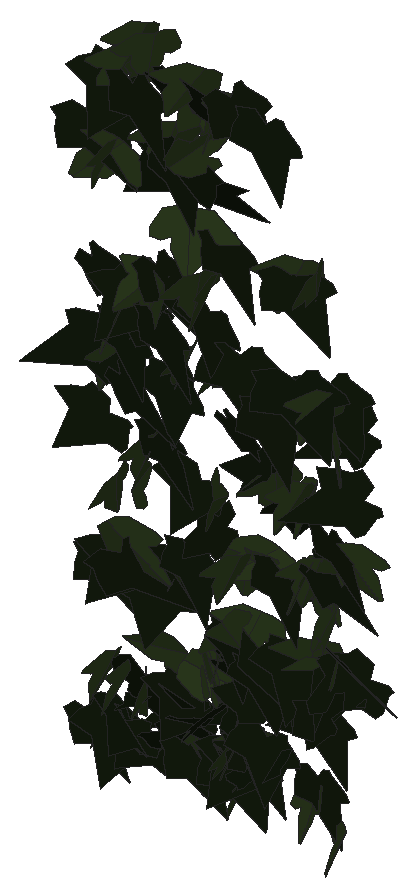
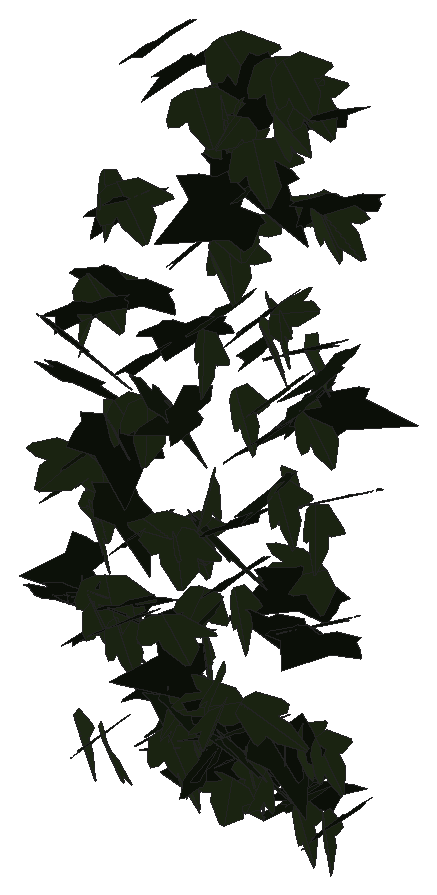
# SketchUp Ruby script. Lengths in inches.
U = 1.inch
M = Sketchup.active_model
def pt(a) = Geom::Point3d.new(a.map { |v| v * U })
def face(e, loops, mat)
  f = e.add_face(loops[0].map { |a| pt(a) })
  loops[1..].each { |l| e.add_face(l.map { |a| pt(a) }).erase! }
  f.material = f.back_material = mat if mat
  f
end
# faces: each face lists its corners as indices into pts; further lists are holes
def faces(e, pts, list, mat = nil) = list.each { |f| face(e, (f[0].is_a?(Array) ? f : [f]).map { |l| l.map { |i| pts[i] } }, mat) }
# xy, xz, yz: faces in a plane at the given z, y or x. An outline is a flat list of corners, or four numbers for a rectangle; further outlines are holes
def ring(l) = l.size == 4 ? [[l[0], l[1]], [l[2], l[1]], [l[2], l[3]], [l[0], l[3]]] : l.each_slice(2).to_a
def flat(e, list, mat, &to3) = list.each { |f| face(e, (f[0].is_a?(Array) ? f : [f]).map { |l| ring(l).map { |u, v| to3.(u, v) } }, mat) }
def xy(e, z, list, mat = nil) = flat(e, list, mat) { |x, y| [x, y, z] }
def xz(e, y, list, mat = nil) = flat(e, list, mat) { |x, z| [x, y, z] }
def yz(e, x, list, mat = nil) = flat(e, list, mat) { |y, z| [x, y, z] }
def lines(e, pts, list) = list.each { |a, b| e.add_line(pt(pts[a]), pt(pts[b])) }
# prism: a flat outline (further loops are holes) pulled along v
def prism(e, loops, v, mat = nil)
  f = face(e, loops, mat); d = Geom::Vector3d.new(v.map { |x| x * U })
  f.pushpull(f.normal.samedirection?(d) ? d.length : -d.length)
end
def box(e, o, s, mat = nil) = prism(e, [[o, [o[0] + s[0], o[1], o[2]], [o[0] + s[0], o[1] + s[1], o[2]], [o[0], o[1] + s[1], o[2]]]], [0, 0, s[2]], mat)
def at(x, y, z, deg = 0) = Geom::Transformation.translation(pt([x, y, z])) * Geom::Transformation.rotation(ORIGIN, Z_AXIS, deg.degrees)
def axes(o, x, y, z) = Geom::Transformation.new([*x, 0, *y, 0, *z, 0, *pt(o).to_a, 1])
def part(name) = M.definitions.add(name)
# library, detail: a bought-in or finely detailed component or shape, given as its bounding box
def library(name, o, s) = part(name).tap { |d| box(d.entities, o, s) }
def detail(e, o, s) = box(e.add_group.entities, o, s)
def put(e, d, t, mat = nil) = e.add_instance(d, t).tap { |i| i.material = mat if mat }
def group(e, t, mat = nil) = e.add_group.tap { |g| g.transformation = t; g.material = mat if mat }.entities
root = M.entities
M.materials.add("1026 AP 7946 SUNNY SIDE UP").color = [254, 231, 186]
M.materials.add("efeu1").color = [18, 25, 13]
M.materials.add("efeu2").color = [43, 57, 29]
c1 = part("ivyleaf_10")
p = [[0,0.5,-0.03],[-0.0625,2.02,-0.43],[-0.19,2.01,-0.46],[-0.54,1.05,-0.29],[-0.52,0.625,-0.18],[-0.83,0.76,-0.28],
  [-1.16,0.64,-0.33],[-1.15,0.33,-0.24],[-0.77,-0.39,0.02],[-0.3,-0.51,0.16],[0.04,-0.48,0.23],[-0.02,2.01,-0.4375],
  [-0.06,2.01,-0.43],[0.04,-0.49,0.23],[0.67,-0.49,0.14],[1.38,0.36,-0.2],[1.375,0.51,-0.24],[0.81,0.65,-0.19],
  [0.62,0.59,-0.15],[0.6,1.09,-0.28],[0.5,1.23,-0.31]]
faces(c1.entities,p,[[0,1,2,3,4,5,6,7,8,9,10],[11,12,0,13,14,15,16,17,18,19,20]],"efeu2")
c2 = part("ivyleaf_9")
p = [[1.54,2.16,1.25],[1.36,2.04,1.19],[-0.21,0.99,0.68],[-0.71,1.11,0.82],[-0.85,0.86,0.67],[-0.8,0.17,0.21],
  [-0.9,-0.01,0.1],[-0.67,-0.16,-0.02],[-0.08,-0.08,-0.05],[-0.03,-0.6,-0.4],[0.65,-0.88,-0.66],[0.83,-0.6,-0.49],
  [1.29,-0.42,-0.43],[1.8125,-0.07,-0.26],[1.21,0.44,0.15]]
faces(c2.entities,p,[[0,1,2,3,4,5,6,7,8,9,10,11,12,13,14]],"efeu1")
put(root,c1,axes([118.05,212.21,283.12],[-0.37131,0.05928,-0.28207],[0.39687,-0.11138,-0.24944],[-0.19234,-0.34425,0.02985]),"1026 AP 7946 SUNNY SIDE UP")
put(root,c2,axes([120.52,212.35,290.41],[0.01109,-0.35714,0.01681],[0.00161,-0.01832,-0.3681],[0.5623,0.00709,0.00072]),"1026 AP 7946 SUNNY SIDE UP")
put(root,c2,axes([120.52,212.35,280.61],[-0.10934,-0.30959,0.0089],[0.00379,-0.01119,-0.32692],[0.48707,-0.06941,0.00454]),"1026 AP 7946 SUNNY SIDE UP")
put(root,c2,axes([118.19,212.31,290.27],[0.13676,-0.35584,-0.02894],[-0.02006,0.02372,-0.37717],[0.56066,0.08765,-0.00644]),"1026 AP 7946 SUNNY SIDE UP")
put(root,c2,axes([117.93,212.4,279.95],[-0.28564,-0.27357,0.00365],[0.01734,-0.01343,-0.33795],[0.42988,-0.18123,0.01606]),"1026 AP 7946 SUNNY SIDE UP")
put(root,c1,axes([121.47,212.29,283.74],[-0.19698,-0.3026,0.06518],[-0.00906,-0.06782,-0.33715],[0.48657,-0.12376,0.02011]),"1026 AP 7946 SUNNY SIDE UP")
put(root,c1,axes([117.95,212.17,283.95],[-0.02269,-0.3263,-0.12185],[0.03595,0.11538,-0.33537],[0.54358,-0.02125,0.01709]),"1026 AP 7946 SUNNY SIDE UP")
put(root,c2,axes([118.17,212.11,282.84],[-0.00464,-0.10566,-0.34058],[0.18482,0.31014,-0.10157],[0.51254,-0.11279,0.03354]),"1026 AP 7946 SUNNY SIDE UP")
put(root,c2,axes([118.06,212.22,285.61],[0.32092,-0.25295,-0.1119],[-0.07031,0.10116,-0.33306],[0.42622,0.20714,0.02932]),"1026 AP 7946 SUNNY SIDE UP")
put(root,c2,axes([117.92,212.5,279.96],[-0.12651,-0.20876,0.23158],[-0.01217,-0.23213,-0.22511],[0.48358,-0.06046,0.05492]),"1026 AP 7946 SUNNY SIDE UP")
put(root,c2,axes([117.8,212.5,290.2],[-0.26607,-0.29238,0.1123],[-0.03521,-0.11418,-0.34671],[0.49031,-0.16686,0.03604]),"1026 AP 7946 SUNNY SIDE UP")
put(root,c2,axes([120.38,212.46,281.5],[-0.05446,-0.29507,0.12324],[0.13746,-0.12612,-0.29108],[0.48245,0.00263,0.09684]),"1026 AP 7946 SUNNY SIDE UP")
put(root,c2,axes([121.09,212.31,286.52],[-0.23251,-0.21185,-0.2599],[0.27253,0.18359,-0.26367],[0.43881,-0.22627,0.02605]),"1026 AP 7946 SUNNY SIDE UP")
put(root,c1,axes([119.45,212.4,287.52],[0.17888,-0.30544,0.1209],[0.04904,-0.1154,-0.33629],[0.51316,0.1175,-0.01]),"1026 AP 7946 SUNNY SIDE UP")
put(root,c1,axes([119.35,212.27,287.6],[-0.16301,-0.33822,-0.0361],[0.0191,0.03091,-0.36424],[0.53402,-0.10435,0.00201]),"1026 AP 7946 SUNNY SIDE UP")
put(root,c1,axes([121.22,212.41,283.57],[0.22591,-0.28506,0.12289],[0.04543,-0.12037,-0.32842],[0.48476,0.14412,-0.02649]),"1026 AP 7946 SUNNY SIDE UP")
put(root,c2,axes([120.6875,212.2,281.27],[-0.45565,-0.12997,0.10381],[0.12293,0.07243,0.32589],[-0.22831,0.29838,-0.03171]),"1026 AP 7946 SUNNY SIDE UP")
put(root,c1,axes([118.5,212.03,284.1],[0.02789,0.02027,0.34666],[-0.25633,0.29534,-0.00775],[-0.46377,-0.16201,0.02514]),"1026 AP 7946 SUNNY SIDE UP")
put(root,c1,axes([119.85,212.34,280.21],[0.09913,-0.30719,0.03282],[0.0014,-0.03412,-0.3232],[0.4859,0.06277,-0.00576]),"1026 AP 7946 SUNNY SIDE UP")
put(root,c2,axes([118.55,212.42,286.56],[0.17204,-0.33683,0.03028],[-0.00069,-0.03304,-0.36488],[0.53191,0.1089,-0.01027]),"1026 AP 7946 SUNNY SIDE UP")
put(root,c2,axes([117.88,212.54,282.48],[-0.30473,-0.22241,0.14591],[-0.02827,-0.16569,-0.29175],[0.41471,-0.17472,0.08733]),"1026 AP 7946 SUNNY SIDE UP")
put(root,c1,axes([118.23,212.55,287.1],[-0.12916,-0.07452,0.33716],[0.07859,-0.3363,-0.06785],[0.52256,0.03216,0.09354]),"1026 AP 7946 SUNNY SIDE UP")
put(root,c2,axes([117.53,212.54,285.94],[-0.01771,-0.10315,-0.36011],[-0.06862,-0.34623,0.10486],[-0.56806,0.04504,-0.00144]),"1026 AP 7946 SUNNY SIDE UP")
put(root,c1,axes([117.79,212.46,286.57],[0.26822,-0.26198,0.14637],[0.08507,-0.1355,-0.32174],[0.46198,0.17705,-0.02574]),"1026 AP 7946 SUNNY SIDE UP")
put(root,c1,axes([121.51,212.43,286.33],[-0.1676,-0.29899,0.14176],[-0.0358,-0.13938,-0.32694],[0.51742,-0.10649,0.0233]),"1026 AP 7946 SUNNY SIDE UP")
put(root,c1,axes([121.84,212.33,279.47],[0.18775,-0.30329,-0.03799],[-0.02193,0.03229,-0.3356],[0.47958,0.12021,-0.00047]),"1026 AP 7946 SUNNY SIDE UP")
put(root,c1,axes([119.2,212.44,290.74],[-0.25116,-0.28206,0.15218],[-0.09781,-0.13627,-0.33451],[0.49221,-0.171,0.01118]),"1026 AP 7946 SUNNY SIDE UP")
put(root,c2,axes([120.53,212.09,280.15],[0.14214,0.19395,0.24319],[-0.13834,0.25126,-0.17733],[-0.45865,-0.01568,0.12885]),"1026 AP 7946 SUNNY SIDE UP")
put(root,c1,axes([119.91,212.41,283.19],[-0.09981,-0.31758,0.06962],[-0.01095,-0.06934,-0.33398],[0.51102,-0.06351,0.00644]),"1026 AP 7946 SUNNY SIDE UP")
put(root,c2,axes([121.43,212.46,281.25],[0.05065,-0.32039,-0.03634],[0.01408,0.0345,-0.33128],[0.50632,0.03109,0.01285]),"1026 AP 7946 SUNNY SIDE UP")
put(root,c2,axes([119.77,212.57,281.8],[0.01605,-0.28926,0.16113],[0.04146,-0.15691,-0.2985],[0.51664,0.02158,0.01895]),"1026 AP 7946 SUNNY SIDE UP")
put(root,c1,axes([117.87,212.51,280.7],[0.09436,-0.26665,0.18193],[0.04982,-0.17539,-0.28252],[0.50175,0.06756,-0.00616]),"1026 AP 7946 SUNNY SIDE UP")
put(root,c2,axes([118.51,212.49,282.375],[-0.36498,-0.20044,-0.10045],[0.14258,0.0419,-0.31453],[0.31933,-0.24781,0.02563]),"1026 AP 7946 SUNNY SIDE UP")
put(root,c2,axes([119.13,212.39,279.96],[0.07979,-0.29118,-0.12477],[0.01211,0.12211,-0.30256],[0.49474,0.04397,0.02753]),"1026 AP 7946 SUNNY SIDE UP")
put(root,c1,axes([117.89,212.5,290.56],[-0.14815,-0.31006,0.15971],[-0.01477,-0.16012,-0.33296],[0.54613,-0.08844,0.03432]),"1026 AP 7946 SUNNY SIDE UP")
put(root,c2,axes([118.13,212.625,279.68],[-0.22099,-0.19114,0.22388],[-0.00666,-0.24129,-0.22177],[0.45632,-0.09609,0.10519]),"1026 AP 7946 SUNNY SIDE UP")
put(root,c2,axes([117.43,212.64,284.62],[-0.34331,-0.18123,0.17849],[-0.07273,-0.19794,-0.27289],[0.38862,-0.19715,0.10661]),"1026 AP 7946 SUNNY SIDE UP")
put(root,c2,axes([121.65,212.32,281.36],[-0.36437,0.21519,0.07506],[-0.09765,0.03829,-0.32525],[-0.343,-0.2395,0.01287]),"1026 AP 7946 SUNNY SIDE UP")
put(root,c1,axes([119.88,212.36,280.22],[0.16901,-0.28456,-0.0873],[-0.03486,0.08046,-0.3128],[0.46484,0.1095,0.00828]),"1026 AP 7946 SUNNY SIDE UP")
put(root,c2,axes([120.47,212.52,285.73],[0.00989,-0.34242,-0.0257],[0.00813,0.0231,-0.35263],[0.53957,0.00593,0.00579]),"1026 AP 7946 SUNNY SIDE UP")
put(root,c2,axes([118.91,212.65,280.59],[-0.24373,-0.23521,0.16587],[0.01614,-0.18915,-0.27332],[0.44909,-0.12085,0.09984]),"1026 AP 7946 SUNNY SIDE UP")
put(root,c2,axes([119.98,212.62,280.01],[-0.32822,-0.22991,0.08729],[-0.03143,-0.09664,-0.31658],[0.38472,-0.20405,0.0486]),"1026 AP 7946 SUNNY SIDE UP")
put(root,c1,axes([120.97,212.52,284.66],[-0.0809,-0.29893,0.14154],[-0.00747,-0.14008,-0.31279],[0.51837,-0.04867,0.01758]),"1026 AP 7946 SUNNY SIDE UP")
put(root,c1,axes([121.62,212.48,285.84],[-0.19204,0.26135,-0.17964],[0.07175,-0.17195,-0.29691],[-0.4901,-0.12758,0.02693]),"1026 AP 7946 SUNNY SIDE UP")
put(root,c2,axes([122.08,212.51,284.92],[-0.50167,0.02603,0.08828],[-0.13906,-0.04512,-0.32593],[-0.02073,-0.32722,0.05]),"1026 AP 7946 SUNNY SIDE UP")
put(root,c2,axes([121.45,212.36,283.69],[0.32651,-0.24493,-0.15128],[-0.07267,0.14864,-0.32496],[0.44198,0.20537,0.05832]),"1026 AP 7946 SUNNY SIDE UP")
put(root,c2,axes([118,212.68,286.68],[-0.32088,-0.22723,0.1565],[-0.04082,-0.17412,-0.3027],[0.42899,-0.18654,0.08826]),"1026 AP 7946 SUNNY SIDE UP")
put(root,c2,axes([119.84,212.53,279.92],[-0.09534,-0.29169,-0.1099],[0.22305,0.06906,-0.28154],[0.43346,-0.09969,0.1207]),"1026 AP 7946 SUNNY SIDE UP")
put(root,c2,axes([119.57,212.42,280.72],[-0.16859,0.26976,-0.13114],[0.05992,-0.12341,-0.29962],[-0.46623,-0.11341,0.00891]),"1026 AP 7946 SUNNY SIDE UP")
put(root,c2,axes([118.77,212.23,280.19],[0.35547,0.17185,0.17006],[0.22571,0.08173,-0.29142],[-0.29775,0.26712,-0.01789]),"1026 AP 7946 SUNNY SIDE UP")
put(root,c2,axes([119,212.6,282.91],[0.01702,-0.32559,0.01876],[-0.00312,-0.02014,-0.33571],[0.51292,0.01068,-0.00266]),"1026 AP 7946 SUNNY SIDE UP")
put(root,c2,axes([119.99,212.65,280.46],[0.02022,-0.30187,0.11982],[0.01947,-0.11757,-0.31187],[0.50927,0.01648,0.00717]),"1026 AP 7946 SUNNY SIDE UP")
put(root,c1,axes([121.55,212.4375,282.92],[0.29415,-0.31004,-0.09883],[-0.06089,0.08657,-0.37236],[0.50586,0.19071,0.01265]),"1026 AP 7946 SUNNY SIDE UP")
put(root,c1,axes([118.48,212.43,287.04],[0.30596,-0.26782,-0.10971],[-0.06688,0.09855,-0.33968],[0.44735,0.19791,0.02425]),"1026 AP 7946 SUNNY SIDE UP")
put(root,c1,axes([119.09,212.3,289.4],[-0.06176,-0.26401,0.26957],[0.10403,0.25549,0.27571],[-0.57684,0.07434,0.02086]),"1026 AP 7946 SUNNY SIDE UP")
put(root,c2,axes([121.47,212.59,284.05],[0.1858,-0.30234,0.05112],[0.02654,-0.04852,-0.33469],[0.48147,0.11935,-0.00128]),"1026 AP 7946 SUNNY SIDE UP")
put(root,c2,axes([118.66,212.67,288.98],[0.0436,-0.31457,0.13948],[0.06484,-0.13358,-0.32492],[0.53571,0.04177,0.02798]),"1026 AP 7946 SUNNY SIDE UP")
put(root,c1,axes([119.24,212.45,280.01],[-0.49317,0.02957,0.00586],[-0.01402,-0.03621,-0.32252],[-0.04517,-0.31159,0.03618]),"1026 AP 7946 SUNNY SIDE UP")
put(root,c1,axes([119.78,212.36,282.15],[-0.14789,-0.2643,-0.18328],[0.14948,0.15215,-0.28616],[0.47677,-0.12969,0.03287]),"1026 AP 7946 SUNNY SIDE UP")
put(root,c2,axes([117.24,212.49,279.83],[0.16529,-0.28242,-0.1147],[-0.03468,0.10871,-0.30936],[0.47515,0.10618,0.01732]),"1026 AP 7946 SUNNY SIDE UP")
put(root,c2,axes([119.88,212.5625,286.39],[-0.1336,-0.30921,-0.13611],[0.07399,0.12218,-0.32941],[0.52244,-0.09637,0.01184]),"1026 AP 7946 SUNNY SIDE UP")
put(root,c1,axes([117.52,212.58,280.76],[0.01132,-0.31376,0.08555],[0.01081,-0.08468,-0.32377],[0.51095,0.00874,0.00495]),"1026 AP 7946 SUNNY SIDE UP")
put(root,c1,axes([119.9375,212.55,279.66],[0.12837,-0.30126,0.03941],[0.00482,-0.04057,-0.32169],[0.47783,0.08134,-0.00735]),"1026 AP 7946 SUNNY SIDE UP")
put(root,c1,axes([118.26,212.43,280.63],[0.12111,-0.2841,-0.12206],[0.0374,0.12564,-0.29776],[0.48158,0.06169,0.05382]),"1026 AP 7946 SUNNY SIDE UP")
put(root,c2,axes([120.55,212.37,285.01],[-0.24553,0.28202,0.08284],[-0.09875,0.05498,-0.33056],[-0.44972,-0.16604,0.02736]),"1026 AP 7946 SUNNY SIDE UP")
put(root,c2,axes([119.21,212.72,286.8125],[-0.03955,-0.30964,0.13812],[0.02479,-0.13713,-0.31984],[0.53109,-0.01666,0.02522]),"1026 AP 7946 SUNNY SIDE UP")
put(root,c2,axes([120.08,212.58,280.24],[0.08954,-0.31135,-0.05016],[0.0424,0.05233,-0.3237],[0.49327,0.05202,0.03693]),"1026 AP 7946 SUNNY SIDE UP")
put(root,c1,axes([120.58,212.47,284.76],[-0.22333,-0.30352,-0.06918],[0.04765,0.05805,-0.34487],[0.48589,-0.1452,0.00203]),"1026 AP 7946 SUNNY SIDE UP")
put(root,c2,axes([117.92,212.61,280.49],[0.12649,-0.08318,0.31169],[0.33278,-0.21687,-0.12048],[0.36524,0.22641,0.00183]),"1026 AP 7946 SUNNY SIDE UP")
put(root,c2,axes([120.84,212.7,281.85],[-0.21586,-0.29723,0.02294],[0.02425,-0.03341,-0.33625],[0.46825,-0.13529,0.02799]),"1026 AP 7946 SUNNY SIDE UP")
put(root,c2,axes([118.58,212.5,290.42],[0.53033,-0.08673,0.09102],[0.12121,-0.05532,-0.35744],[0.15304,0.34437,-0.0323]),"1026 AP 7946 SUNNY SIDE UP")
put(root,c1,axes([117.53,212.61,288.96],[0.06499,-0.34102,0.04491],[-0.00603,-0.04631,-0.35403],[0.54095,0.04046,-0.00934]),"1026 AP 7946 SUNNY SIDE UP")
put(root,c1,axes([118.98,212.57,288.28],[0.45725,0.23068,-0.0269],[-0.00602,-0.03917,-0.38151],[-0.36522,0.28945,-0.02739]),"1026 AP 7946 SUNNY SIDE UP")
put(root,c2,axes([120.5,212.69,283.11],[0.04967,-0.33154,0.02036],[-0.01163,-0.02244,-0.34309],[0.52229,0.03103,-0.00958]),"1026 AP 7946 SUNNY SIDE UP")
put(root,c1,axes([117.61,212.54,288.97],[0.46329,0.03142,-0.19936],[-0.30853,0.043,-0.30004],[-0.00368,0.34997,0.05685]),"1026 AP 7946 SUNNY SIDE UP")
put(root,c2,axes([117.67,212.72,286.04],[0.08519,-0.32724,0.07468],[0.01551,-0.07372,-0.34213],[0.52743,0.05502,-0.002]),"1026 AP 7946 SUNNY SIDE UP")
put(root,c1,axes([118.75,212.55,280.16],[0.11894,-0.30593,-0.05773],[-0.02078,0.05267,-0.32435],[0.48812,0.07679,0.00026]),"1026 AP 7946 SUNNY SIDE UP")
put(root,c1,axes([117.66,212.65,285.75],[-0.07557,-0.32514,0.09445],[-0.01155,-0.09344,-0.33909],[0.53186,-0.04823,0.00605]),"1026 AP 7946 SUNNY SIDE UP")
put(root,c1,axes([117.99,212.68,290.92],[-0.1207,-0.32944,0.13102],[-0.00027,-0.13202,-0.34807],[0.55635,-0.07154,0.02825]),"1026 AP 7946 SUNNY SIDE UP")
put(root,c2,axes([120.8,212.6,287.98],[0.02529,-0.31507,-0.16094],[0.02139,0.15504,-0.32349],[0.55132,0.00844,0.01994]),"1026 AP 7946 SUNNY SIDE UP")
put(root,c2,axes([118.85,212.58,289.21],[0.19246,0.04176,-0.35801],[-0.44639,-0.20394,-0.12935],[-0.32258,0.30713,-0.0346]),"1026 AP 7946 SUNNY SIDE UP")
put(root,c2,axes([121.32,212.74,281.7],[-0.36774,-0.19647,-0.11015],[0.22973,-0.01897,-0.29652],[0.26521,-0.25599,0.10412]),"1026 AP 7946 SUNNY SIDE UP")
put(root,c2,axes([117.61,212.6,282.48],[-0.15109,-0.23597,-0.21671],[0.17642,0.17861,-0.25981],[0.46322,-0.14499,0.02827]),"1026 AP 7946 SUNNY SIDE UP")
put(root,c2,axes([119.76,212.56,290.49],[0.13787,-0.29304,-0.18817],[-0.03183,0.18206,-0.3127],[0.54064,0.08545,0.02957]),"1026 AP 7946 SUNNY SIDE UP")
put(root,c1,axes([119.35,212.55,290.09],[0.23529,-0.29505,-0.13108],[-0.04686,0.12517,-0.33885],[0.50202,0.14997,0.02981]),"1026 AP 7946 SUNNY SIDE UP")
put(root,c1,axes([121.16,212.73,283.3],[-0.28298,0.11519,-0.26024],[0.22809,-0.21855,-0.20987],[-0.37333,-0.22084,0.06904]),"1026 AP 7946 SUNNY SIDE UP")
put(root,c2,axes([120.91,212.83,281.56],[-0.15873,-0.28705,0.1064],[-0.00006,-0.11048,-0.31208],[0.48056,-0.09482,0.03511]),"1026 AP 7946 SUNNY SIDE UP")
put(root,c1,axes([120.99,212.73,284.59],[0.29268,-0.25712,0.1076],[0.07834,-0.09454,-0.32723],[0.43017,0.19216,-0.01361]),"1026 AP 7946 SUNNY SIDE UP")
put(root,c1,axes([120.8,212.71,288.09],[-0.29027,-0.27182,0.11971],[-0.03401,-0.126,-0.33533],[0.46455,-0.17907,0.05025]),"1026 AP 7946 SUNNY SIDE UP")
put(root,c2,axes([119.5,212.68,283.5],[-0.44664,0.14683,-0.06215],[0.05375,-0.06591,-0.32693],[-0.24426,-0.28299,0.04171]),"1026 AP 7946 SUNNY SIDE UP")
put(root,c2,axes([121.43,212.67,282.17],[0.38976,-0.19453,0.08859],[0.11147,-0.05074,-0.32488],[0.31605,0.25779,0.00533]),"1026 AP 7946 SUNNY SIDE UP")
put(root,c2,axes([117.14,212.67,289.31],[-0.01807,-0.29801,-0.19195],[0.12835,0.17737,-0.29914],[0.53608,-0.05252,0.06515]),"1026 AP 7946 SUNNY SIDE UP")
put(root,c1,axes([119.52,212.5625,281.66],[0.17823,-0.26133,-0.15668],[-0.03669,0.15281,-0.29036],[0.47285,0.11036,0.03653]),"1026 AP 7946 SUNNY SIDE UP")
put(root,c1,axes([118.15,212.68,284.41],[-0.02726,-0.33196,0.00953],[0.00446,-0.01129,-0.34249],[0.52224,-0.01723,0.00342]),"1026 AP 7946 SUNNY SIDE UP")
put(root,c1,axes([118.97,212.39,289.84],[-0.00805,-0.11694,-0.34866],[0.1002,0.33211,-0.1175],[0.55305,-0.06187,0.01621]),"1026 AP 7946 SUNNY SIDE UP")
put(root,c1,axes([117.4,212.65,279.68],[0.11696,-0.30092,-0.03721],[0.04445,0.04218,-0.31677],[0.47418,0.07027,0.03888]),"1026 AP 7946 SUNNY SIDE UP")
put(root,c1,axes([119.54,212.54,286.21],[-0.00162,-0.29138,-0.18262],[0.00944,0.17557,-0.29911],[0.53486,-0.00398,0.00473]),"1026 AP 7946 SUNNY SIDE UP")
put(root,c1,axes([117.81,212.68,279.7],[0.06759,-0.31802,-0.01566],[-0.00358,0.01321,-0.33052],[0.50049,0.04304,-0.00025]),"1026 AP 7946 SUNNY SIDE UP")
put(root,c1,axes([118.22,212.68,290.86],[-0.25772,-0.32189,-0.00101],[0.02459,-0.00891,-0.37171],[0.50555,-0.16366,0.01756]),"1026 AP 7946 SUNNY SIDE UP")
put(root,c1,axes([120.97,212.81,279.6875],[0.34994,-0.21236,0.13086],[0.11509,-0.10839,-0.31643],[0.37271,0.23286,-0.02516]),"1026 AP 7946 SUNNY SIDE UP")
put(root,c1,axes([120.22,212.75,283.3],[0.35644,0.07999,-0.2287],[-0.33392,-0.06651,-0.24796],[-0.16332,0.31056,0.00783]),"1026 AP 7946 SUNNY SIDE UP")
put(root,c2,axes([119.625,212.7,285.21],[0.37564,-0.24391,-0.01445],[0.02705,0.03444,-0.34952],[0.38308,0.23674,0.03885]),"1026 AP 7946 SUNNY SIDE UP")
put(root,c1,axes([121.15,212.63,288.1],[0.0384,-0.32782,-0.11605],[0.0398,0.11246,-0.33641],[0.54266,0.01495,0.03288]),"1026 AP 7946 SUNNY SIDE UP")
put(root,c1,axes([118.53,212.73,289.52],[-0.25802,-0.30485,0.03981],[-0.00596,-0.04375,-0.35647],[0.4835,-0.16322,0.01685]),"1026 AP 7946 SUNNY SIDE UP")
put(root,c2,axes([118.31,212.52,280.45],[-0.0109,0.30942,0.05313],[-0.12552,0.04644,-0.30834],[-0.47654,-0.01931,0.08]),"1026 AP 7946 SUNNY SIDE UP")
put(root,c2,axes([118.31,212.7,287.24],[0.19218,-0.29555,-0.13324],[-0.04377,0.12634,-0.32803],[0.50432,0.12359,0.02231]),"1026 AP 7946 SUNNY SIDE UP")
put(root,c2,axes([119.37,212.8125,279.92],[0.25345,-0.25768,0.09104],[0.05261,-0.08489,-0.31318],[0.42586,0.16385,-0.01549]),"1026 AP 7946 SUNNY SIDE UP")
put(root,c1,axes([119.46,212.49,284.04],[0.04365,-0.15056,-0.31285],[0.00246,0.3039,-0.15373],[0.53177,0.01096,0.02639]),"1026 AP 7946 SUNNY SIDE UP")
put(root,c1,axes([119.96,212.7,283.17],[-0.48586,-0.0879,0.05733],[-0.0752,-0.03663,-0.3304],[0.14576,-0.31191,0.02065]),"1026 AP 7946 SUNNY SIDE UP")
put(root,c2,axes([119.42,212.8,287.95],[0.13012,-0.33224,-0.0519],[-0.03591,0.04426,-0.35228],[0.52673,0.08509,-0.0112]),"1026 AP 7946 SUNNY SIDE UP")
put(root,c2,axes([118.85,212.95,283.9],[-0.21033,-0.26493,0.13276],[-0.03821,-0.13277,-0.30439],[0.46271,-0.13139,0.03521]),"1026 AP 7946 SUNNY SIDE UP")
put(root,c2,axes([121.89,212.88,281.81],[-0.47072,-0.09306,0.07523],[-0.08911,-0.0632,-0.32037],[0.16385,-0.30172,0.04189]),"1026 AP 7946 SUNNY SIDE UP")
put(root,c2,axes([118.22,212.81,284.5],[0.18981,-0.31161,-0.01241],[-0.014,0.00757,-0.34417],[0.49004,0.12091,-0.00503]),"1026 AP 7946 SUNNY SIDE UP")
put(root,c1,axes([121.3,212.8125,281.85],[0.30254,-0.25122,0.07226],[0.06362,-0.05915,-0.32631],[0.40578,0.19658,-0.00271]),"1026 AP 7946 SUNNY SIDE UP")
put(root,c1,axes([119,212.76,279.75],[-0.48891,0.03133,-0.03896],[0.03998,-0.10584,-0.30493],[-0.06632,-0.29482,0.10336]),"1026 AP 7946 SUNNY SIDE UP")
put(root,c2,axes([119.85,212.74,280.73],[-0.35291,0.22518,-0.02213],[-0.06954,-0.07507,-0.31629],[-0.34901,-0.21273,0.0854]),"1026 AP 7946 SUNNY SIDE UP")
put(root,c1,axes([120.79,212.79,281.51],[-0.0789,-0.31776,0.03576],[-0.00919,-0.03605,-0.33162],[0.50284,-0.05052,-0.00045]),"1026 AP 7946 SUNNY SIDE UP")
put(root,c1,axes([121.05,212.83,281.74],[-0.18252,-0.28517,0.09753],[0.00235,-0.10375,-0.31529],[0.47327,-0.10947,0.03918]),"1026 AP 7946 SUNNY SIDE UP")
put(root,c1,axes([121.03,212.77,282.07],[-0.36249,-0.22382,0.04678],[-0.02614,-0.0497,-0.33039],[0.35855,-0.2299,0.0232]),"1026 AP 7946 SUNNY SIDE UP")
put(root,c1,axes([119.9,212.83,280.18],[-0.2403,-0.26152,0.09458],[-0.01486,-0.10153,-0.30974],[0.43635,-0.14748,0.04154]),"1026 AP 7946 SUNNY SIDE UP")
put(root,c2,axes([121.3,212.8125,286.32],[-0.02157,-0.31023,-0.13564],[0.08056,0.12656,-0.31622],[0.52267,-0.03231,0.04314]),"1026 AP 7946 SUNNY SIDE UP")
put(root,c1,axes([117.9,212.94,290.32],[0.08766,-0.28292,0.20254],[0.05873,-0.19467,-0.2982],[0.53999,0.0671,-0.00045]),"1026 AP 7946 SUNNY SIDE UP")
put(root,c1,axes([118.81,212.76,282.64],[0.0561,-0.32264,-0.04905],[0.01484,0.04706,-0.33381],[0.51219,0.03398,0.01504]),"1026 AP 7946 SUNNY SIDE UP")
put(root,c1,axes([121.64,212.74,283.8125],[-0.4671,-0.01988,-0.15562],[0.2392,-0.02521,-0.30514],[0.0098,-0.33226,0.03051]),"1026 AP 7946 SUNNY SIDE UP")
put(root,c2,axes([121.02,212.89,279.91],[0.08989,-0.30795,0.003],[0.00126,-0.00459,-0.3227],[0.48428,0.05717,0.00028]),"1026 AP 7946 SUNNY SIDE UP")
put(root,c2,axes([120.9375,212.66,284.44],[0.19295,0.28797,-0.10926],[-0.05146,-0.10306,-0.32292],[-0.48068,0.12663,-0.00929]),"1026 AP 7946 SUNNY SIDE UP")
put(root,c2,axes([118.375,212.98,285.3125],[-0.04924,-0.31726,0.08951],[-0.01283,-0.08832,-0.32894],[0.51783,-0.03236,0.00036]),"1026 AP 7946 SUNNY SIDE UP")
put(root,c2,axes([120.875,212.66,283.43],[-0.06857,0.32232,-0.00901],[-0.03118,-0.01333,-0.33443],[-0.50613,-0.04284,0.02182]),"1026 AP 7946 SUNNY SIDE UP")
put(root,c2,axes([121.875,212.84,285.78],[-0.49006,0.12594,0.02165],[-0.04884,-0.02294,-0.34477],[-0.19454,-0.31148,0.03202]),"1026 AP 7946 SUNNY SIDE UP")
put(root,c1,axes([119.18,212.75,281.33],[-0.11902,0.31544,-0.00281],[-0.00851,-0.00594,-0.33415],[-0.49597,-0.07559,0.00641]),"1026 AP 7946 SUNNY SIDE UP")
put(root,c2,axes([118.87,212.85,280.47],[-0.43661,0.1427,-0.05027],[0.03513,-0.06388,-0.31848],[-0.23495,-0.27474,0.04581]),"1026 AP 7946 SUNNY SIDE UP")
put(root,c2,axes([119.52,212.76,281.3],[0.45363,-0.01936,0.15162],[0.2261,-0.04441,-0.29643],[0.05867,0.32086,-0.02995]),"1026 AP 7946 SUNNY SIDE UP")
put(root,c1,axes([118.42,212.83,280.13],[-0.39549,0.17449,-0.07145],[0.05525,-0.07182,-0.31334],[-0.29062,-0.25111,0.03767]),"1026 AP 7946 SUNNY SIDE UP")
put(root,c1,axes([118.19,212.92,286.95],[0.28,-0.28458,0.03036],[0.00734,-0.03372,-0.34573],[0.45007,0.17759,-0.01325]),"1026 AP 7946 SUNNY SIDE UP")
put(root,c1,axes([119.35,212.95,290.125],[-0.34156,-0.25782,0.09124],[0.01889,-0.12395,-0.33654],[0.42899,-0.19982,0.08747]),"1026 AP 7946 SUNNY SIDE UP")
put(root,c1,axes([119.86,212.97,282],[-0.41462,-0.13346,0.11788],[-0.04928,-0.16845,-0.27597],[0.27279,-0.23328,0.12931]),"1026 AP 7946 SUNNY SIDE UP")
put(root,c1,axes([119,212.74,281.04],[0.15774,0.10823,0.2973],[0.34682,0.18585,-0.15002],[-0.33721,0.24177,-0.01523]),"1026 AP 7946 SUNNY SIDE UP")
put(root,c2,axes([117.0625,212.85,286.875],[0.31187,-0.2557,-0.11364],[-0.04038,0.1163,-0.32895],[0.4351,0.19407,0.05092]),"1026 AP 7946 SUNNY SIDE UP")
put(root,c1,axes([118.48,212.8125,281.11],[0.16485,0.01589,-0.30997],[-0.43502,0.13151,-0.09136],[0.18804,0.29032,0.0604]),"1026 AP 7946 SUNNY SIDE UP")
put(root,c2,axes([117.85,212.93,286.29],[0.23652,-0.27542,-0.12536],[-0.02725,0.12616,-0.31961],[0.47167,0.1454,0.0444]),"1026 AP 7946 SUNNY SIDE UP")
put(root,c1,axes([119.89,212.7,280.6],[0.00682,0.02729,0.32959],[-0.20924,0.29118,-0.02204],[-0.45923,-0.13227,0.01494]),"1026 AP 7946 SUNNY SIDE UP")
put(root,c1,axes([119.08,212.93,280.93],[-0.01004,0.31699,-0.0028],[0.00289,-0.00448,-0.32665],[-0.49848,-0.00641,-0.00184]),"1026 AP 7946 SUNNY SIDE UP")
put(root,c1,axes([118.59,212.99,285.85],[0.0222,-0.33186,-0.02646],[-0.01649,0.02337,-0.34191],[0.5229,0.01482,-0.00966]),"1026 AP 7946 SUNNY SIDE UP")
put(root,c2,axes([118.79,212.86,288.69],[0.50752,0.08746,0.09206],[0.13127,0.03157,-0.34421],[-0.14561,0.33329,0.01055]),"1026 AP 7946 SUNNY SIDE UP")
